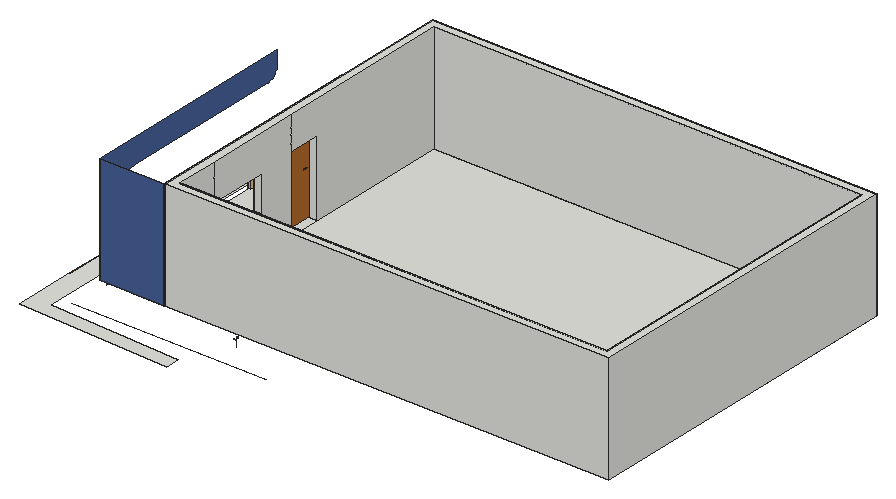
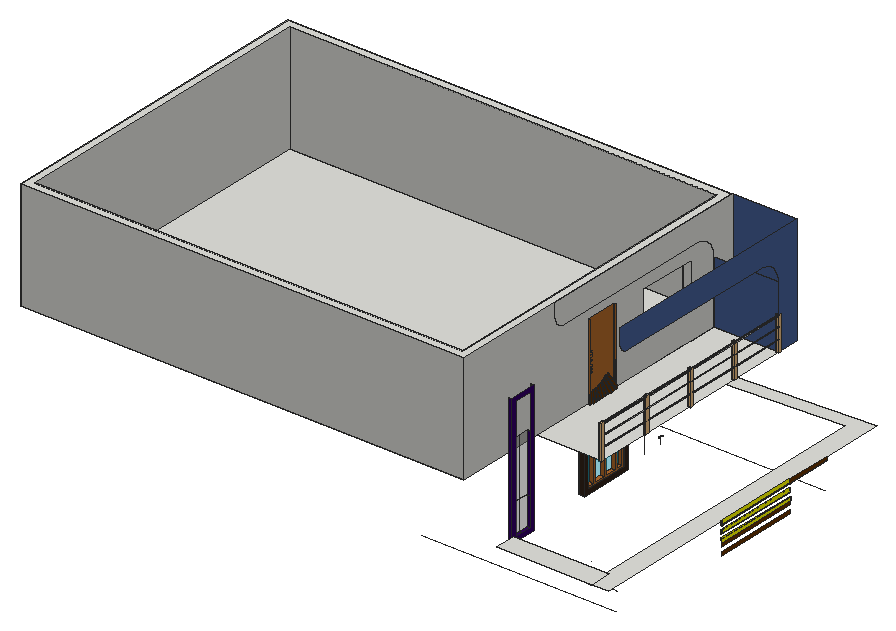
# SketchUp Ruby script. Lengths in inches.
U = 1.inch
M = Sketchup.active_model
def pt(a) = Geom::Point3d.new(a.map { |v| v * U })
def face(e, loops, mat)
  f = e.add_face(loops[0].map { |a| pt(a) })
  loops[1..].each { |l| e.add_face(l.map { |a| pt(a) }).erase! }
  f.material = f.back_material = mat if mat
  f
end
# faces: each face lists its corners as indices into pts; further lists are holes
def faces(e, pts, list, mat = nil) = list.each { |f| face(e, (f[0].is_a?(Array) ? f : [f]).map { |l| l.map { |i| pts[i] } }, mat) }
# xy, xz, yz: faces in a plane at the given z, y or x. An outline is a flat list of corners, or four numbers for a rectangle; further outlines are holes
def ring(l) = l.size == 4 ? [[l[0], l[1]], [l[2], l[1]], [l[2], l[3]], [l[0], l[3]]] : l.each_slice(2).to_a
def flat(e, list, mat, &to3) = list.each { |f| face(e, (f[0].is_a?(Array) ? f : [f]).map { |l| ring(l).map { |u, v| to3.(u, v) } }, mat) }
def xy(e, z, list, mat = nil) = flat(e, list, mat) { |x, y| [x, y, z] }
def xz(e, y, list, mat = nil) = flat(e, list, mat) { |x, z| [x, y, z] }
def yz(e, x, list, mat = nil) = flat(e, list, mat) { |y, z| [x, y, z] }
def lines(e, pts, list) = list.each { |a, b| e.add_line(pt(pts[a]), pt(pts[b])) }
# prism: a flat outline (further loops are holes) pulled along v
def prism(e, loops, v, mat = nil)
  f = face(e, loops, mat); d = Geom::Vector3d.new(v.map { |x| x * U })
  f.pushpull(f.normal.samedirection?(d) ? d.length : -d.length)
end
def box(e, o, s, mat = nil) = prism(e, [[o, [o[0] + s[0], o[1], o[2]], [o[0] + s[0], o[1] + s[1], o[2]], [o[0], o[1] + s[1], o[2]]]], [0, 0, s[2]], mat)
def at(x, y, z, deg = 0) = Geom::Transformation.translation(pt([x, y, z])) * Geom::Transformation.rotation(ORIGIN, Z_AXIS, deg.degrees)
def axes(o, x, y, z) = Geom::Transformation.new([*x, 0, *y, 0, *z, 0, *pt(o).to_a, 1])
def part(name) = M.definitions.add(name)
# library, detail: a bought-in or finely detailed component or shape, given as its bounding box
def library(name, o, s) = part(name).tap { |d| box(d.entities, o, s) }
def detail(e, o, s) = box(e.add_group.entities, o, s)
def put(e, d, t, mat = nil) = e.add_instance(d, t).tap { |i| i.material = mat if mat }
def group(e, t, mat = nil) = e.add_group.tap { |g| g.transformation = t; g.material = mat if mat }.entities
root = M.entities
M.materials.add("Teddy_HairLight").color = [51, 36, 26]
M.materials.add("[Color C08]").color = [102, 51, 0]
M.materials.add("[Color E05]").color = [255, 255, 0]
M.materials.add("[Color J08]").color = [51, 0, 102]
M.materials.add("[Formica Blue]").color = [71, 97, 152]
M.materials.add("[Translucent Glass Gray]").color = [128, 128, 128]
M.materials["[Translucent Glass Gray]"].alpha = 0.5
M.materials.add("[Translucent Glass Tinted]").color = [8, 201, 241]
M.materials["[Translucent Glass Tinted]"].alpha = 0.48
M.materials.add("[Wood Bamboo]").color = [177, 105, 43]
c1 = part("Group11\#1")
xz(c1.entities,-529.44,[[54.75,137.61,54.85,137.62,54.95,137.66,55.03,137.72,55.09,137.8,55.13,137.9,55.14,138,55.13,138.1,55.09,138.2,55.03,138.28,54.95,138.34,54.85,138.38,54.75,138.39,54.65,138.38,54.55,138.34,54.47,138.28,54.41,138.2,54.37,138.1,54.36,138,54.37,137.9,54.41,137.8,54.47,137.72,54.55,137.66,54.65,137.62],[54.75,149.61,54.85,149.62,54.95,149.66,55.03,149.72,55.09,149.8,55.13,149.9,55.14,150,55.13,150.1,55.09,150.2,55.03,150.28,54.95,150.34,54.85,150.38,54.75,150.39,54.65,150.38,54.55,150.34,54.47,150.28,54.41,150.2,54.37,150.1,54.36,150,54.37,149.9,54.41,149.8,54.47,149.72,54.55,149.66,54.65,149.62],[54.75,161.21,54.95,161.24,55.14,161.32,55.31,161.44,55.43,161.61,55.51,161.8,55.54,162,55.51,162.2,55.43,162.39,55.31,162.56,55.14,162.68,54.95,162.76,54.75,162.79,54.55,162.76,54.36,162.68,54.19,162.56,54.07,162.39,53.99,162.2,53.96,162,53.99,161.8,54.07,161.61,54.19,161.44,54.36,161.32,54.55,161.24]])
xz(c1.entities,-285.65,[[54.75,137.61,54.65,137.62,54.55,137.66,54.47,137.72,54.41,137.8,54.37,137.9,54.36,138,54.37,138.1,54.41,138.2,54.47,138.28,54.55,138.34,54.65,138.38,54.75,138.39,54.85,138.38,54.95,138.34,55.03,138.28,55.09,138.2,55.13,138.1,55.14,138,55.13,137.9,55.09,137.8,55.03,137.72,54.95,137.66,54.85,137.62],[54.75,149.61,54.65,149.62,54.55,149.66,54.47,149.72,54.41,149.8,54.37,149.9,54.36,150,54.37,150.1,54.41,150.2,54.47,150.28,54.55,150.34,54.65,150.38,54.75,150.39,54.85,150.38,54.95,150.34,55.03,150.28,55.09,150.2,55.13,150.1,55.14,150,55.13,149.9,55.09,149.8,55.03,149.72,54.95,149.66,54.85,149.62],[54.75,161.21,54.55,161.24,54.36,161.32,54.19,161.44,54.07,161.61,53.99,161.8,53.96,162,53.99,162.2,54.07,162.39,54.19,162.56,54.36,162.68,54.55,162.76,54.75,162.79,54.95,162.76,55.14,162.68,55.31,162.56,55.43,162.39,55.51,162.2,55.54,162,55.51,161.8,55.43,161.61,55.31,161.44,55.14,161.32,54.95,161.24]])
p = [[54.75,-468.49,137.61],[54.75,-529.44,137.61],[54.65,-529.44,137.62],[54.65,-468.49,137.62],[54.65,-407.54,137.62],[54.65,-346.59,137.62],
  [54.65,-285.65,137.62],[54.75,-285.65,137.61],[54.75,-346.59,137.61],[54.75,-407.54,137.61],[54.55,-529.44,137.66],[54.55,-468.49,137.66],
  [54.55,-407.54,137.66],[54.55,-346.59,137.66],[54.55,-285.65,137.66],[54.85,-468.49,137.62],[54.85,-529.44,137.62],[54.85,-285.65,137.62],
  [54.85,-346.59,137.62],[54.85,-407.54,137.62],[54.95,-468.49,137.66],[54.95,-529.44,137.66],[54.95,-285.65,137.66],[54.95,-346.59,137.66],
  [54.95,-407.54,137.66],[54.47,-346.59,137.72],[54.47,-407.54,137.72],[54.47,-468.49,137.72],[54.47,-529.44,137.72],[54.41,-529.44,137.8],
  [54.41,-468.49,137.8],[54.41,-407.54,137.8],[54.41,-346.59,137.8],[54.41,-285.65,137.8],[54.47,-285.65,137.72],[55.03,-468.49,137.72],
  [55.03,-529.44,137.72],[55.03,-285.65,137.72],[55.03,-346.59,137.72],[55.03,-407.54,137.72],[55.09,-468.49,137.8],[55.09,-529.44,137.8],
  [55.09,-285.65,137.8],[55.09,-346.59,137.8],[55.09,-407.54,137.8],[54.37,-285.65,137.9],[54.37,-529.44,137.9],[54.37,-468.49,137.9],
  [54.37,-407.54,137.9],[54.37,-346.59,137.9],[55.13,-468.49,137.9],[55.13,-529.44,137.9],[55.13,-285.65,137.9],[55.13,-346.59,137.9],
  [55.13,-407.54,137.9],[54.36,-285.65,138],[54.36,-529.44,138],[54.36,-468.49,138],[54.36,-407.54,138],[54.36,-346.59,138],
  [55.14,-468.49,138],[55.14,-529.44,138],[55.14,-285.65,138],[55.14,-346.59,138],[55.14,-407.54,138],[54.37,-529.44,138.1],
  [54.37,-468.49,138.1],[54.37,-407.54,138.1],[54.37,-346.59,138.1],[54.37,-285.65,138.1],[55.13,-468.49,138.1],[55.13,-529.44,138.1],
  [55.13,-285.65,138.1],[55.13,-346.59,138.1],[55.13,-407.54,138.1],[54.41,-529.44,138.2],[54.41,-468.49,138.2],[54.41,-407.54,138.2],
  [54.41,-346.59,138.2],[54.41,-285.65,138.2],[55.09,-468.49,138.2],[55.09,-529.44,138.2],[55.09,-285.65,138.2],[55.09,-346.59,138.2],
  [55.09,-407.54,138.2],[54.47,-529.44,138.28],[54.47,-468.49,138.28],[54.47,-407.54,138.28],[54.47,-346.59,138.28],[54.47,-285.65,138.28],
  [55.03,-468.49,138.28],[55.03,-529.44,138.28],[55.03,-285.65,138.28],[55.03,-346.59,138.28],[55.03,-407.54,138.28],[54.55,-529.44,138.34],
  [54.55,-468.49,138.34],[54.55,-407.54,138.34],[54.55,-346.59,138.34],[54.55,-285.65,138.34],[54.65,-529.44,138.38],[54.65,-468.49,138.38],
  [54.65,-407.54,138.38],[54.65,-346.59,138.38],[54.65,-285.65,138.38],[54.95,-468.49,138.34],[54.95,-529.44,138.34],[54.95,-285.65,138.34],
  [54.95,-346.59,138.34],[54.95,-407.54,138.34],[54.85,-468.49,138.38],[54.85,-529.44,138.38],[54.85,-285.65,138.38],[54.85,-346.59,138.38],
  [54.85,-407.54,138.38],[54.75,-529.44,138.39],[54.75,-468.49,138.39],[54.75,-407.54,138.39],[54.75,-346.59,138.39],[54.75,-285.65,138.39],
  [54.55,-285.65,149.66],[54.65,-285.65,149.62],[54.65,-346.59,149.62],[54.65,-407.54,149.62],[54.65,-468.49,149.62],[54.65,-529.44,149.62],
  [54.55,-529.44,149.66],[54.55,-468.49,149.66],[54.55,-407.54,149.66],[54.55,-346.59,149.66],[54.75,-285.65,149.61],[54.75,-346.59,149.61],
  [54.75,-407.54,149.61],[54.75,-468.49,149.61],[54.75,-529.44,149.61],[54.85,-346.59,149.62],[54.85,-407.54,149.62],[54.85,-468.49,149.62],
  [54.85,-529.44,149.62],[54.85,-285.65,149.62],[54.95,-468.49,149.66],[54.95,-529.44,149.66],[54.95,-285.65,149.66],[54.95,-346.59,149.66],
  [54.95,-407.54,149.66],[54.41,-285.65,149.8],[54.47,-285.65,149.72],[54.47,-346.59,149.72],[54.47,-407.54,149.72],[54.47,-468.49,149.72],
  [54.47,-529.44,149.72],[54.41,-529.44,149.8],[54.41,-468.49,149.8],[54.41,-407.54,149.8],[54.41,-346.59,149.8],[55.03,-468.49,149.72],
  [55.03,-529.44,149.72],[55.03,-285.65,149.72],[55.03,-346.59,149.72],[55.03,-407.54,149.72],[55.09,-468.49,149.8],[55.09,-529.44,149.8],
  [55.09,-285.65,149.8],[55.09,-346.59,149.8],[55.09,-407.54,149.8],[54.37,-285.65,149.9],[54.37,-529.44,149.9],[54.37,-468.49,149.9],
  [54.37,-407.54,149.9],[54.37,-346.59,149.9],[55.13,-468.49,149.9],[55.13,-529.44,149.9],[55.13,-285.65,149.9],[55.13,-346.59,149.9],
  [55.13,-407.54,149.9],[54.36,-529.44,150],[54.36,-468.49,150],[54.36,-407.54,150],[54.36,-346.59,150],[54.36,-285.65,150],
  [55.14,-468.49,150],[55.14,-529.44,150],[55.14,-285.65,150],[55.14,-346.59,150],[55.14,-407.54,150],[54.37,-529.44,150.1],
  [54.37,-468.49,150.1],[54.37,-407.54,150.1],[54.37,-346.59,150.1],[54.37,-285.65,150.1],[55.13,-468.49,150.1],[55.13,-529.44,150.1],
  [55.13,-285.65,150.1],[55.13,-346.59,150.1],[55.13,-407.54,150.1],[54.41,-529.44,150.2],[54.41,-468.49,150.2],[54.41,-407.54,150.2],
  [54.41,-346.59,150.2],[54.41,-285.65,150.2],[55.09,-468.49,150.2],[55.09,-529.44,150.2],[55.09,-285.65,150.2],[55.09,-346.59,150.2],
  [55.09,-407.54,150.2],[54.47,-529.44,150.28],[54.47,-468.49,150.28],[54.47,-407.54,150.28],[54.47,-346.59,150.28],[54.47,-285.65,150.28],
  [55.03,-468.49,150.28],[55.03,-529.44,150.28],[55.03,-285.65,150.28],[55.03,-346.59,150.28],[55.03,-407.54,150.28],[54.55,-529.44,150.34],
  [54.55,-468.49,150.34],[54.55,-407.54,150.34],[54.55,-346.59,150.34],[54.55,-285.65,150.34],[54.65,-529.44,150.38],[54.65,-468.49,150.38],
  [54.65,-407.54,150.38],[54.65,-346.59,150.38],[54.65,-285.65,150.38],[54.95,-468.49,150.34],[54.95,-529.44,150.34],[54.95,-285.65,150.34],
  [54.95,-346.59,150.34],[54.95,-407.54,150.34],[54.85,-468.49,150.38],[54.85,-529.44,150.38],[54.85,-285.65,150.38],[54.85,-346.59,150.38],
  [54.85,-407.54,150.38],[54.75,-529.44,150.39],[54.75,-468.49,150.39],[54.75,-407.54,150.39],[54.75,-346.59,150.39],[54.75,-285.65,150.39],
  [54.55,-346.59,161.24],[54.55,-407.54,161.24],[54.55,-468.49,161.24],[54.55,-529.44,161.24],[54.36,-529.44,161.32],[54.36,-468.49,161.32],
  [54.36,-407.54,161.32],[54.36,-346.59,161.32],[54.36,-285.65,161.32],[54.55,-285.65,161.24],[54.75,-285.65,161.21],[54.75,-346.59,161.21],
  [54.75,-407.54,161.21],[54.75,-468.49,161.21],[54.75,-529.44,161.21],[54.95,-346.59,161.24],[54.95,-407.54,161.24],[54.95,-468.49,161.24],
  [54.95,-529.44,161.24],[54.95,-285.65,161.24],[55.14,-346.59,161.32],[55.14,-407.54,161.32],[55.14,-468.49,161.32],[55.14,-529.44,161.32],
  [55.14,-285.65,161.32],[54.19,-529.44,161.44],[54.19,-468.49,161.44],[54.19,-407.54,161.44],[54.19,-346.59,161.44],[54.19,-285.65,161.44],
  [55.31,-285.65,161.44],[55.31,-346.59,161.44],[55.31,-407.54,161.44],[55.31,-468.49,161.44],[55.31,-529.44,161.44],[54.07,-285.65,161.61],
  [54.07,-529.44,161.61],[54.07,-468.49,161.61],[54.07,-407.54,161.61],[54.07,-346.59,161.61],[55.43,-468.49,161.61],[55.43,-529.44,161.61],
  [55.43,-285.65,161.61],[55.43,-346.59,161.61],[55.43,-407.54,161.61],[53.99,-285.65,161.8],[53.99,-529.44,161.8],[53.99,-468.49,161.8],
  [53.99,-407.54,161.8],[53.99,-346.59,161.8],[55.51,-468.49,161.8],[55.51,-529.44,161.8],[55.51,-285.65,161.8],[55.51,-346.59,161.8],
  [55.51,-407.54,161.8],[53.96,-529.44,162],[53.96,-468.49,162],[53.96,-407.54,162],[53.96,-346.59,162],[53.96,-285.65,162],
  [55.54,-468.49,162],[55.54,-529.44,162],[55.54,-285.65,162],[55.54,-346.59,162],[55.54,-407.54,162],[53.99,-529.44,162.2],
  [53.99,-468.49,162.2],[53.99,-407.54,162.2],[53.99,-346.59,162.2],[53.99,-285.65,162.2],[55.51,-468.49,162.2],[55.51,-529.44,162.2],
  [55.51,-285.65,162.2],[55.51,-346.59,162.2],[55.51,-407.54,162.2],[54.07,-529.44,162.39],[54.07,-468.49,162.39],[54.07,-407.54,162.39],
  [54.07,-346.59,162.39],[54.07,-285.65,162.39],[55.43,-468.49,162.39],[55.43,-529.44,162.39],[55.43,-285.65,162.39],[55.43,-346.59,162.39],
  [55.43,-407.54,162.39],[54.19,-529.44,162.56],[54.19,-468.49,162.56],[54.19,-407.54,162.56],[54.19,-346.59,162.56],[54.19,-285.65,162.56],
  [55.31,-468.49,162.56],[55.31,-529.44,162.56],[55.31,-285.65,162.56],[55.31,-346.59,162.56],[55.31,-407.54,162.56],[54.36,-529.44,162.68],
  [54.36,-468.49,162.68],[54.36,-407.54,162.68],[54.36,-346.59,162.68],[54.36,-285.65,162.68],[55.14,-468.49,162.68],[55.14,-529.44,162.68],
  [55.14,-285.65,162.68],[55.14,-346.59,162.68],[55.14,-407.54,162.68],[54.55,-529.44,162.76],[54.55,-468.49,162.76],[54.55,-407.54,162.76],
  [54.55,-346.59,162.76],[54.55,-285.65,162.76],[54.95,-468.49,162.76],[54.95,-529.44,162.76],[54.95,-285.65,162.76],[54.95,-346.59,162.76],
  [54.95,-407.54,162.76],[54.75,-529.44,162.79],[54.75,-468.49,162.79],[54.75,-407.54,162.79],[54.75,-346.59,162.79],[54.75,-285.65,162.79]]
faces(c1.entities,p,[[0,1,2,3,4,5,6,7,8,9],[5,4,3,2,10,11,12,13,14,6],[15,16,1,0,9,8,7,17,18,19],[20,21,16,15,19,18,17,22,23,24],[25,26,27,28,29,30,31,32,33,34],[13,12,11,10,28,27,26,25,34,14],[35,36,21,20,24,23,22,37,38,39],[40,41,36,35,39,38,37,42,43,44],
  [45,33,32,31,30,29,46,47,48,49],[50,51,41,40,44,43,42,52,53,54],[55,45,49,48,47,46,56,57,58,59],[60,61,51,50,54,53,52,62,63,64],[57,56,65,66,67,68,69,55,59,58],[70,71,61,60,64,63,62,72,73,74],[66,65,75,76,77,78,79,69,68,67],[80,81,71,70,74,73,72,82,83,84],
  [76,75,85,86,87,88,89,79,78,77],[90,91,81,80,84,83,82,92,93,94],[86,85,95,96,97,98,99,89,88,87],[96,95,100,101,102,103,104,99,98,97],[105,106,91,90,94,93,92,107,108,109],[110,111,106,105,109,108,107,112,113,114],[101,100,115,116,117,118,119,104,103,102],[116,115,111,110,114,113,112,119,118,117],
  [120,121,122,123,124,125,126,127,128,129],[121,130,131,132,133,134,125,124,123,122],[135,136,137,138,134,133,132,131,130,139],[140,141,138,137,136,135,139,142,143,144],[145,146,147,148,149,150,151,152,153,154],[146,120,129,128,127,126,150,149,148,147],[155,156,141,140,144,143,142,157,158,159],[160,161,156,155,159,158,157,162,163,164],
  [165,145,154,153,152,151,166,167,168,169],[170,171,161,160,164,163,162,172,173,174],[167,166,175,176,177,178,179,165,169,168],[180,181,171,170,174,173,172,182,183,184],[176,175,185,186,187,188,189,179,178,177],[190,191,181,180,184,183,182,192,193,194],[186,185,195,196,197,198,199,189,188,187],[200,201,191,190,194,193,192,202,203,204],
  [196,195,205,206,207,208,209,199,198,197],[210,211,201,200,204,203,202,212,213,214],[206,205,215,216,217,218,219,209,208,207],[216,215,220,221,222,223,224,219,218,217],[225,226,211,210,214,213,212,227,228,229],[230,231,226,225,229,228,227,232,233,234],[221,220,235,236,237,238,239,224,223,222],[236,235,231,230,234,233,232,239,238,237],
  [240,241,242,243,244,245,246,247,248,249],[249,250,251,252,253,254,243,242,241,240],[255,256,257,258,254,253,252,251,250,259],[260,261,262,263,258,257,256,255,259,264],[247,246,245,244,265,266,267,268,269,248],[264,270,271,272,273,274,263,262,261,260],[275,269,268,267,266,265,276,277,278,279],[280,281,274,273,272,271,270,282,283,284],
  [285,275,279,278,277,276,286,287,288,289],[290,291,281,280,284,283,282,292,293,294],[287,286,295,296,297,298,299,285,289,288],[300,301,291,290,294,293,292,302,303,304],[296,295,305,306,307,308,309,299,298,297],[310,311,301,300,304,303,302,312,313,314],[306,305,315,316,317,318,319,309,308,307],[320,321,311,310,314,313,312,322,323,324],
  [316,315,325,326,327,328,329,319,318,317],[330,331,321,320,324,323,322,332,333,334],[326,325,335,336,337,338,339,329,328,327],[340,341,331,330,334,333,332,342,343,344],[336,335,345,346,347,348,349,339,338,337],[350,351,341,340,344,343,342,352,353,354],[346,345,355,356,357,358,359,349,348,347],[356,355,351,350,354,353,352,359,358,357]])
c2 = library("Ploe\#1",[53.18,-287.22,126],[3.14,3.15,37.57])
c3 = part("Group10\#1")
put(c3.entities,c2,at(0,0,0))
put(c3.entities,c2,at(0,-60.95,0))
put(c3.entities,c2,at(0,-121.9,0))
put(c3.entities,c2,at(0,-182.85,0))
put(c3.entities,c2,at(0,-243.8,0))
xy(root,42,[[203,150.79,209,165.8125],[203,165.8125,209,188.27],[203,188.27,209,210.79]],"Teddy_HairLight")
xy(root,46.18,[[205,154.97,209,161.63],[205,161.63,209,184.09],[205,184.09,209,206.61]])
xy(root,46.18,[[203,154.97,205,161.63],[203,161.63,205,184.09],[203,184.09,205,206.61]],"Teddy_HairLight")
xy(root,47.34,[[205,195.84,209,205.53]],"[Wood Bamboo]")
xy(root,47.75,[[205,165.79,209,178.97],[205,180.97,209,194.16]],"[Wood Bamboo]")
xy(root,48.01,[[205,156.48,209,164.16]],"[Wood Bamboo]")
xy(root,57.69,[[182,306.65,185,336.96]])
xy(root,62.42,[[182,311.38,185,321.81],[182,321.81,185,332.23]],"[Color J08]")
xy(root,71.76,[[68.66,345.83,173,369.14]])
xy(root,78.26,[[205,156.48,209,164.16]],"[Wood Bamboo]")
xy(root,78.4375,[[205,165.79,209,178.97],[205,180.97,209,194.16]],"[Wood Bamboo]")
xy(root,78.59,[[205,195.84,209,205.53]],"[Wood Bamboo]")
xy(root,79.82,[[205,154.97,209,206.61]])
xy(root,79.82,[[203,154.97,205,206.61]],"Teddy_HairLight")
xy(root,84,[[203,150.79,209,165.76],[203,165.76,209,188.27],[203,188.27,209,210.79]],"Teddy_HairLight")
xy(root,126,[[137.625,0.14,208.5625,25.13],[137.625,25.13,137.625,268.93,208.5625,268.93,208.5625,198.98,206.625,198.98,206.625,162.98,208.5625,162.98,208.5625,25.13]])
xy(root,126,[[206.625,162.98,208.5625,198.98],[208.5625,162.98,209,198.98]],"[Wood Bamboo]")
xy(root,126.02,[[205.5,165.63,206.625,168.26],[205.625,170.59,206.625,173.61],[205.625,176.55,206.625,178.7],[205.625,180.98,206.625,182.01],[205.625,182.01,206.625,183.03],
  [205.625,185.07,206.625,186.09],[205.625,186.09,206.625,187.12],[205.625,189.16,206.625,190.18],[205.625,190.18,206.625,191.2],[205.625,193.15,206.625,195.09],
  [205.625,196.8,206.625,198.97]],"[Wood Bamboo]")
xz(root,0.14,[[137.625,126,208.5625,246]],"[Formica Blue]")
xz(root,25.13,[[137.625,126,208.5625,194.81]],"[Formica Blue]")
xz(root,119.2,[[50.21,51.11,49.21,51.15,49.37,55.4,50.37,55.36],[50.53,59.63,49.53,59.67,49.68,63.93,50.68,63.89],[50.84,68.16,49.84,68.19,50,72.45,51,72.41]])
xz(root,150.79,[[203,42,209,84]],"Teddy_HairLight")
xz(root,154.97,[[205,46.18,209,79.82]])
xz(root,154.97,[[203,46.18,205,79.82]],"Teddy_HairLight")
xz(root,156.48,[[205,48.01,209,78.26]],"[Wood Bamboo]")
xz(root,162.98,[[206.625,126,209,210]],"[Wood Bamboo]")
xz(root,163,[[205.625,126.02,206.625,130.19]],"[Wood Bamboo]")
xz(root,164.16,[[205,48.01,209,78.26]],"[Wood Bamboo]")
xz(root,165.79,[[205,47.75,209,78.4375]],"[Wood Bamboo]")
xz(root,178.97,[[205,47.75,209,78.4375]],"[Wood Bamboo]")
xz(root,180.97,[[205,47.75,209,78.4375]],"[Wood Bamboo]")
xz(root,194.16,[[205,47.75,209,78.4375]],"[Wood Bamboo]")
xz(root,195.84,[[205,47.34,209,78.59]],"[Wood Bamboo]")
xz(root,198.97,[[205.625,126.02,206.625,136.14]],"[Wood Bamboo]")
xz(root,198.98,[[206.625,126,206.625,158.03,204.625,158.03,204.625,159.65,206.625,159.65,206.625,161.11,204.625,161.11,204.625,162.48,206.625,162.48,206.625,164.59,204.625,164.59,204.625,165.85,206.625,165.85,206.625,170.15,204.625,170.15,204.625,171.41,206.625,171.41,206.625,173.52,204.625,173.52,204.625,174.89,206.625,174.89,206.625,176.35,204.625,176.35,204.625,177.97,206.625,177.97,206.625,210,209,210,209,126]],"[Wood Bamboo]")
xz(root,205.53,[[205,47.34,209,78.59]],"[Wood Bamboo]")
xz(root,206.61,[[205,46.18,209,79.82]])
xz(root,206.61,[[203,46.18,205,79.82]],"[Wood Bamboo]")
xz(root,210.79,[[203,42,209,84]],"Teddy_HairLight")
xz(root,213.24,[[50.53,59.63,50.68,63.89,49.68,63.93,49.53,59.67],[50.84,68.16,51,72.41,50,72.45,49.84,68.19]])
xz(root,306.65,[[182,57.69,185,201.38]],"[Color J08]")
xz(root,311.38,[[182,62.42,185,94.23],[182,94.23,185,157.72]],"[Color J08]")
xz(root,332.23,[[182,62.42,185,94.23],[182,94.23,185,157.72]],"[Color J08]")
xz(root,336.96,[[182,57.69,185,201.38]],"[Color J08]")
yz(root,49.84,[[68.0625,68.1875,119.2,68.19],[119.2,68.1875,213.24,68.19]])
yz(root,137.625,[[0.14,126,0.14,246,244.43,246,244.43,232.56,244.32,230.81,243.98,229.08,243.41,227.42,242.63,225.84,241.66,224.38,240.5,223.06,239.18,221.9,237.71,220.92,236.14,220.14,234.47,219.58,232.75,219.24,230.99,219.12,49.45,219.12,46.27,218.91,43.15,218.29,40.14,217.27,37.29,215.86,34.64,214.1,32.25,212,30.16,209.61,28.39,206.96,26.98,204.11,25.96,201.1,25.34,197.98,25.13,194.81,25.13,126]],"[Formica Blue]")
yz(root,182,[[[306.65,57.69,336.96,201.38],[311.38,62.42,332.23,196.65]]],"[Color J08]")
yz(root,185,[[311.38,62.42,321.81,94.23],[321.81,62.42,332.23,94.23],[311.38,94.23,321.81,157.72],[321.81,94.23,332.23,157.72]],"[Translucent Glass Gray]")
yz(root,203,[[[150.79,42,210.79,84],[154.97,46.18,206.61,79.82]]],"Teddy_HairLight")
yz(root,205,[[[154.97,46.18,206.61,79.82],[180.97,47.75,194.16,78.4375],[165.79,47.75,178.97,78.4375],[195.84,47.34,205.53,78.59],[156.48,48.01,164.16,78.26]]],"[Wood Bamboo]")
yz(root,205.5,[[165.63,126.02,178.05,145.21,179.7,144.06,168.26,126.02]],"[Color C08]")
yz(root,205.625,[[163,126.02,163,130.19,175.42,147.03,176.73,146.12],[170.59,126.02,181.2,143.02,182.1875,142.33,173.61,126.02],[176.55,126.02,183.08,141.7,184.02,141.05,178.7,126.02],[180.98,126.02,184.88,140.45,185.85,140.23,186.81,140.02,183.03,126.02],[185.07,126.02,188.25,139.69,188.74,139.58,189.7,139.36,190.66,139.15,187.12,126.02],
  [189.16,126.02,192.59,138.71,193.55,138.49,191.2,126.02],[193.15,126.02,194.52,138.27,196.125,137.91,195.09,126.02],[196.8,126.02,197.55,138.14,198.97,138.38,198.97,126.02]],"[Color C08]")
yz(root,206.625,[[162.98,126,162.98,154.9,163,154.91,163,126.02,182.01,126.02,182,126],[182,126,182.01,126.02,183.03,126.02,183.02,126],[183.02,126,183.03,126.02,184.05,126.02,184.05,126],[184.05,126,185.07,126.02],[185.07,126,186.09,126.02],
  [186.09,126,186.09,126.02,187.12,126.02,187.11,126],[187.11,126,187.12,126.02,188.14,126.02,188.13,126],[188.13,126,188.14,126.02,189.16,126.02,189.16,126],[189.16,126,190.18,126.02],[190.18,126,191.2,126.02],
  [191.2,126,195.09,126.02],[195.09,126,195.09,126.02,198.97,126.02,198.97,136.14,198.98,136.14,198.98,126],[163,126.02,176.73,146.12,178.05,145.21,165.63,126.02],[168.26,126.02,179.7,144.06,181.2,143.02,170.59,126.02],[173.61,126.02,182.1875,142.33,183.08,141.7,176.55,126.02],
  [178.7,126.02,184.02,141.05,184.88,140.45,180.98,126.02],[183.03,126.02,186.81,140.02,188.25,139.69,185.07,126.02],[187.12,126.02,190.66,139.15,192.59,138.71,189.16,126.02],[191.2,126.02,193.55,138.49,194.52,138.27,193.15,126.02],[195.09,126.02,196.125,137.91,197.55,138.14,196.8,126.02]],"[Wood Bamboo]")
yz(root,208.5625,[[0.14,126,25.13,126,25.13,194.81,25.34,197.98,25.96,201.1,26.98,204.11,28.39,206.96,30.16,209.61,32.25,212,34.64,214.1,37.29,215.86,40.14,217.27,43.15,218.29,46.27,218.91,49.45,219.12,230.99,219.12,232.75,219.24,234.47,219.58,236.14,220.14,237.71,220.92,239.18,221.9,240.5,223.06,241.66,224.38,242.63,225.84,243.41,227.42,243.98,229.08,244.32,230.81,244.43,232.56,244.43,246,0.14,246]])
yz(root,209,[[150.79,42,165.76,42,165.76,46.18,154.97,46.18,154.97,79.82,165.76,79.82,165.76,84,150.79,84],[165.76,42,188.27,46.18],[188.27,42,210.79,42,210.79,84,188.27,84,188.27,79.82,206.61,79.82,206.61,46.18,188.27,46.18],[165.76,79.82,188.27,84]])
yz(root,209,[[195.84,47.34,205.53,78.59],[165.79,47.75,178.97,78.4375],[180.97,47.75,188.27,78.4375],[188.27,47.75,194.16,78.4375],[156.48,48.01,164.16,78.26]],"[Translucent Glass Tinted]")
yz(root,209,[[[162.98,126,198.98,210],[197.03,175.09,196.76,175.13,196.54,175.22,190.72,175.22,190.72,177.09,196.54,177.09,196.76,177.18,197.03,177.22,197.31,177.18,197.5625,177.07,197.78,176.91,197.95,176.6875,198.06,176.43,198.1,176.15,198.06,175.88,197.95,175.625,197.78,175.4,197.5625,175.23,197.31,175.13]]],"[Wood Bamboo]")
p = [[49.89,213.24,42.58],[49.74,213.24,38.32],[49.74,119.2,38.32],[49.89,119.2,42.58],[50.21,213.24,51.1],[50.05,213.24,46.85],
  [50.05,119.2,46.85],[50.21,119.2,51.1],[50.37,213.24,55.36],[50.21,213.24,51.11],[50.21,119.2,51.11],[50.37,119.2,55.36],
  [49.37,119.2,55.4],[49.37,213.24,55.4],[49.53,213.24,59.67],[49.53,119.2,59.67],[50.53,119.2,59.63],[50.53,213.24,59.63],
  [50.68,213.24,63.89],[50.68,119.2,63.89],[49.68,119.2,63.93],[49.68,213.24,63.93],[211.6875,15.24,66.45],[71.32,15.24,71.66],
  [71.32,369.14,71.66],[68.94,369.14,71.75],[68.66,369.14,71.76],[50,369.14,72.45],[50,213.24,72.45],[51,213.24,72.41],
  [51,119.2,72.41],[50,119.2,72.45],[50,68.0625,72.45],[50,0.14,72.45],[211.6875,0.14,66.45],[49.84,119.2,68.19],
  [49.84,68.0625,68.19],[49.84,213.24,68.19],[50.84,119.2,68.16],[50.84,213.24,68.16],[206.625,176.73,146.12],[206.625,163,126.02],
  [205.625,163,126.02],[205.625,176.73,146.12],[206.625,165.63,126.02],[206.625,178.05,145.21],[205.5,178.05,145.21],[205.5,165.63,126.02],
  [206.625,179.7,144.06],[206.625,168.26,126.02],[205.5,168.26,126.02],[205.5,179.7,144.06],[206.625,170.59,126.02],[206.625,181.2,143.02],
  [205.625,181.2,143.02],[205.625,170.59,126.02],[206.625,182.1875,142.33],[206.625,173.61,126.02],[205.625,173.61,126.02],[205.625,182.1875,142.33],
  [206.625,176.55,126.02],[206.625,183.08,141.7],[205.625,183.08,141.7],[205.625,176.55,126.02],[206.625,184.02,141.05],[206.625,178.7,126.02],
  [205.625,178.7,126.02],[205.625,184.02,141.05],[206.625,180.98,126.02],[206.625,184.88,140.45],[205.625,184.88,140.45],[205.625,180.98,126.02],
  [206.625,186.81,140.02],[206.625,183.03,126.02],[205.625,183.03,126.02],[205.625,186.81,140.02],[206.625,185.07,126.02],[206.625,188.25,139.69],
  [205.625,188.25,139.69],[205.625,185.07,126.02],[206.625,190.66,139.15],[206.625,187.12,126.02],[205.625,187.12,126.02],[205.625,190.66,139.15],
  [206.625,189.16,126.02],[206.625,192.59,138.71],[205.625,192.59,138.71],[205.625,189.16,126.02],[206.625,193.55,138.49],[206.625,191.2,126.02],
  [205.625,191.2,126.02],[205.625,193.55,138.49],[206.625,193.15,126.02],[206.625,194.52,138.27],[205.625,194.52,138.27],[205.625,193.15,126.02],
  [206.625,196.125,137.91],[206.625,195.09,126.02],[205.625,195.09,126.02],[205.625,196.125,137.91],[206.625,196.8,126.02],[206.625,197.55,138.14],
  [205.625,197.55,138.14],[205.625,196.8,126.02],[209,103.97,126],[209,67.97,126],[209,100.76,50.66],[207.5,100.76,50.66],
  [209,100.81,50.6875],[207.5,100.81,50.6875],[209,100.97,50.76],[207.5,100.97,50.76],[209,101.15,50.78],[207.5,101.15,50.78],
  [209,101.33,50.76],[207.5,101.33,50.76],[209,101.49,50.6875],[207.5,101.49,50.6875],[209,101.64,50.58],[207.5,101.64,50.58],
  [209,101.75,50.4375],[207.5,101.75,50.4375],[209,101.82,50.27],[207.5,101.82,50.27],[209,101.84,50.09],[207.5,101.84,50.09],
  [209,101.82,49.92],[207.5,101.82,49.92],[209,101.75,49.75],[207.5,101.75,49.75],[209,101.64,49.61],[207.5,101.64,49.61],
  [209,101.49,49.5],[207.5,101.49,49.5],[209,101.33,49.43],[207.5,101.33,49.43],[209,101.15,49.41],[207.5,101.15,49.41],
  [209,100.97,49.43],[207.5,100.97,49.43],[209,100.81,49.5],[207.5,100.81,49.5],[209,100.76,49.53],[207.5,100.76,49.53],
  [209,97.21,49.53],[207.5,97.21,49.53],[209,97.21,50.66],[207.5,97.21,50.66],[206.625,182,126],[206.625,181.95,125.8],
  [206.625,183.02,126],[206.625,182.91,125.58],[206.625,184.05,126],[206.625,183.875,125.36],[206.625,185.07,126],[206.625,184.84,125.15],
  [206.625,186.09,126],[206.625,185.8,124.93],[206.625,187.11,126],[206.625,186.76,124.71],[206.625,188.13,126],[206.625,187.73,124.49],
  [206.625,189.16,126],[206.625,188.6875,124.28],[206.625,190.18,126],[206.625,189.65,124.06],[206.625,191.2,126],[206.625,190.62,123.84],
  [68.66,369.14,94.84],[68.59,369.14,94.84],[209,188.27,47.75],[209,188.27,46.18],[209,188.27,79.82],[209,188.27,78.4375],
  [209,165.76,79.82],[209,165.76,46.18],[209,143.25,84],[209,143.25,42],[203,143.25,84],[209,120.74,84],
  [209,120.74,42],[203,120.74,84],[209,98.22,49.53],[209,98.22,42],[209,98.22,50.66],[207.5,98.22,84],
  [203,98.22,84],[209,183.02,47.34],[205,183.02,47.34],[209,160.56,47.34],[205,160.56,47.34],[49.99,366.4,72.14],
  [49.96,363.76,71.3125],[49.91,361.33,70.01],[49.85,359.1875,68.27],[49.77,357.41,66.16],[49.07,359.35,47.36],[264.26,359.35,47.36],
  [48.82,71.87,40.75],[264.01,71.87,40.75]]
faces(root,p,[[0,1,2,3],[4,5,6,7],[31,35,36,32]],"[Color C08]")
faces(root,p,[[8,9,10,11],[18,17,16,19],[29,39,38,30]],"[Color E05]")
faces(root,p,[[12,13,8,11],[14,15,16,17],[20,21,18,19],[22,23,24,25,26,27,28,29,30,31,32,33,34],[37,35,38,39]])
faces(root,p,[[40,41,42,43],[44,45,46,47],[48,49,50,51],[52,53,54,55],[56,57,58,59],[60,61,62,63],[64,65,66,67],[68,69,70,71],
  [72,73,74,75],[76,77,78,79],[80,81,82,83],[84,85,86,87],[88,89,90,91],[92,93,94,95],[96,97,98,99],[100,101,102,103]],"[Wood Bamboo]")
lines(root,p,[[104,105],[106,107],[108,109],[110,111],[112,113],[114,115],[116,117],[118,119],[120,121],[122,123],[124,125],[126,127],
  [128,129],[130,131],[132,133],[134,135],[136,137],[138,139],[140,141],[142,143],[144,145],[146,147],[148,149],[150,151],
  [152,153],[154,155],[156,157],[158,159],[160,161],[162,163],[164,165],[166,167],[168,169],[170,171],[172,173],[174,175],
  [176,177],[176,178],[179,180],[179,181],[182,183],[184,182],[185,186],[187,188],[189,190],[27,191],[191,192],[192,193],
  [193,194],[194,195],[196,197],[198,199]])
g1 = group(root,at(136.05,23.56,126))
put(g1,c1,at(-53.18,531.02,-126))
put(g1,c3,at(-53.18,531.02,-126))
g2 = group(root,at(209,0.14,126))
xy(g2,0,[[0,0,489,0,489,369,0,369,0,198.85,9,198.85,9,360,480,360,480,9,9,9,9,56.04,0,56.04],[9,9,480,360],[0,150.65,9,162.85],[0,162.85,9,198.85]])
xy(g2,40.26,[[0,56.04,9,122.56]])
xy(g2,79.74,[[0,56.04,9,122.56]])
xy(g2,84,[[0,162.85,9,198.85]])
xy(g2,120,[[[0,0,489,369],[9,9,480,360]]])
xz(g2,0,[[0,0,489,120]])
xz(g2,9,[[9,0,480,120]])
xz(g2,56.04,[[0,40.26,9,79.74]])
xz(g2,122.56,[[0,40.26,9,79.74]])
xz(g2,162.85,[[0,0,9,84]])
xz(g2,198.85,[[0,0,9,84]])
xz(g2,360,[[9,0,480,120]])
xz(g2,369,[[0,0,489,120]])
yz(g2,0,[[[0,0,0,120,369,120,369,0,198.85,0,198.85,84,162.85,84,162.85,0],[56.04,40.26,122.56,79.74]]])
yz(g2,9,[[9,0,56.04,120],[56.04,0,162.85,0,162.85,120,56.04,120,56.04,79.74,122.56,79.74,122.56,40.26,56.04,40.26],[198.85,0,360,0,360,120,162.85,120,162.85,84,198.85,84]])
yz(g2,480,[[9,0,360,120]])
yz(g2,489,[[0,0,369,120]])
